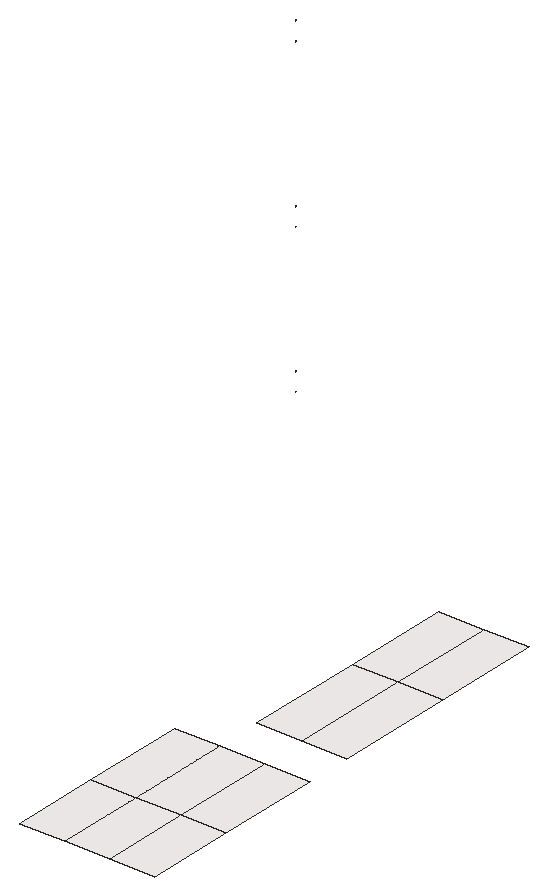
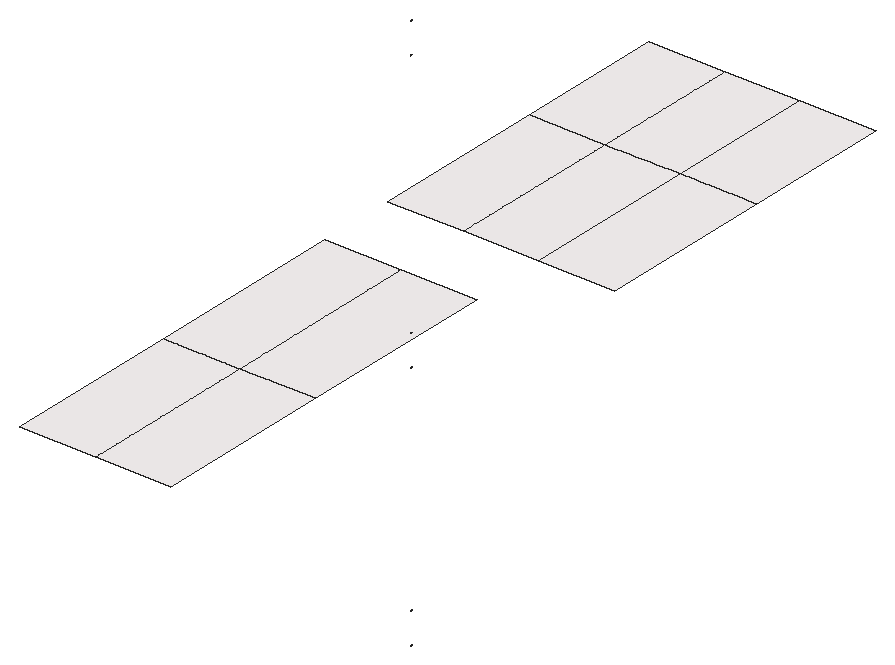
# SketchUp Ruby script. Lengths in inches.
U = 1.inch
M = Sketchup.active_model
def pt(a) = Geom::Point3d.new(a.map { |v| v * U })
def face(e, loops, mat)
  f = e.add_face(loops[0].map { |a| pt(a) })
  loops[1..].each { |l| e.add_face(l.map { |a| pt(a) }).erase! }
  f.material = f.back_material = mat if mat
  f
end
# faces: each face lists its corners as indices into pts; further lists are holes
def faces(e, pts, list, mat = nil) = list.each { |f| face(e, (f[0].is_a?(Array) ? f : [f]).map { |l| l.map { |i| pts[i] } }, mat) }
# xy, xz, yz: faces in a plane at the given z, y or x. An outline is a flat list of corners, or four numbers for a rectangle; further outlines are holes
def ring(l) = l.size == 4 ? [[l[0], l[1]], [l[2], l[1]], [l[2], l[3]], [l[0], l[3]]] : l.each_slice(2).to_a
def flat(e, list, mat, &to3) = list.each { |f| face(e, (f[0].is_a?(Array) ? f : [f]).map { |l| ring(l).map { |u, v| to3.(u, v) } }, mat) }
def xy(e, z, list, mat = nil) = flat(e, list, mat) { |x, y| [x, y, z] }
def xz(e, y, list, mat = nil) = flat(e, list, mat) { |x, z| [x, y, z] }
def yz(e, x, list, mat = nil) = flat(e, list, mat) { |y, z| [x, y, z] }
def lines(e, pts, list) = list.each { |a, b| e.add_line(pt(pts[a]), pt(pts[b])) }
# prism: a flat outline (further loops are holes) pulled along v
def prism(e, loops, v, mat = nil)
  f = face(e, loops, mat); d = Geom::Vector3d.new(v.map { |x| x * U })
  f.pushpull(f.normal.samedirection?(d) ? d.length : -d.length)
end
def box(e, o, s, mat = nil) = prism(e, [[o, [o[0] + s[0], o[1], o[2]], [o[0] + s[0], o[1] + s[1], o[2]], [o[0], o[1] + s[1], o[2]]]], [0, 0, s[2]], mat)
def at(x, y, z, deg = 0) = Geom::Transformation.translation(pt([x, y, z])) * Geom::Transformation.rotation(ORIGIN, Z_AXIS, deg.degrees)
def axes(o, x, y, z) = Geom::Transformation.new([*x, 0, *y, 0, *z, 0, *pt(o).to_a, 1])
def part(name) = M.definitions.add(name)
# library, detail: a bought-in or finely detailed component or shape, given as its bounding box
def library(name, o, s) = part(name).tap { |d| box(d.entities, o, s) }
def detail(e, o, s) = box(e.add_group.entities, o, s)
def put(e, d, t, mat = nil) = e.add_instance(d, t).tap { |i| i.material = mat if mat }
def group(e, t, mat = nil) = e.add_group.tap { |g| g.transformation = t; g.material = mat if mat }.entities
root = M.entities
M.materials.add("Material \#1").color = [140, 140, 140]
M.materials.add("[0010_Snow]").color = [255, 250, 250]
c1 = part("3DGeom~8_Defintion")
xz(c1.entities,-471.94,[[458.125,-17.29,459.53,-16.11,457.73,-17.15],[458.125,-17.29,458.54,-17.29,459.53,-16.11],[458.54,-17.29,458.93,-17.15,459.53,-16.11],[457.73,-17.15,459.53,-16.11,457.42,-16.88],[458.93,-17.15,459.25,-16.88,459.53,-16.11],
  [457.42,-16.88,459.53,-16.11,457.21,-16.52],[459.25,-16.88,459.46,-16.52,459.53,-16.11],[457.21,-16.52,459.53,-16.11,457.14,-16.11],[457.14,-16.11,459.53,-16.11,457.21,-15.7],[459.53,-16.11,457.42,-15.34,457.21,-15.7],
  [459.53,-16.11,457.73,-15.07,457.42,-15.34],[459.53,-16.11,458.125,-14.93,457.73,-15.07],[459.53,-16.11,458.54,-14.93,458.125,-14.93],[459.53,-16.11,458.93,-15.07,458.54,-14.93],[459.53,-16.11,459.25,-15.34,458.93,-15.07],
  [459.53,-16.11,459.46,-15.7,459.25,-15.34]],"Material \#1")
xz(c1.entities,-416.39,[[458.125,-17.29,457.73,-17.15,459.53,-16.11],[458.125,-17.29,459.53,-16.11,458.54,-17.29],[458.54,-17.29,459.53,-16.11,458.93,-17.15],[457.73,-17.15,457.42,-16.88,459.53,-16.11],[458.93,-17.15,459.53,-16.11,459.25,-16.88],
  [457.42,-16.88,457.21,-16.52,459.53,-16.11],[459.25,-16.88,459.53,-16.11,459.46,-16.52],[457.21,-16.52,457.14,-16.11,459.53,-16.11],[457.14,-16.11,457.21,-15.7,459.53,-16.11],[459.53,-16.11,457.21,-15.7,457.42,-15.34],
  [459.53,-16.11,457.42,-15.34,457.73,-15.07],[459.53,-16.11,457.73,-15.07,458.125,-14.93],[459.53,-16.11,458.125,-14.93,458.54,-14.93],[459.53,-16.11,458.54,-14.93,458.93,-15.07],[459.53,-16.11,458.93,-15.07,459.25,-15.34],
  [459.53,-16.11,459.25,-15.34,459.46,-15.7]],"Material \#1")
xz(c1.entities,-27.5,[[458.125,-17.29,459.53,-16.11,457.73,-17.15],[458.125,-17.29,458.54,-17.29,459.53,-16.11],[458.54,-17.29,458.93,-17.15,459.53,-16.11],[457.73,-17.15,459.53,-16.11,457.42,-16.88],[458.93,-17.15,459.25,-16.88,459.53,-16.11],
  [457.42,-16.88,459.53,-16.11,457.21,-16.52],[459.25,-16.88,459.46,-16.52,459.53,-16.11],[457.21,-16.52,459.53,-16.11,457.14,-16.11],[457.14,-16.11,459.53,-16.11,457.21,-15.7],[459.53,-16.11,457.42,-15.34,457.21,-15.7],
  [459.53,-16.11,457.73,-15.07,457.42,-15.34],[459.53,-16.11,458.125,-14.93,457.73,-15.07],[459.53,-16.11,458.54,-14.93,458.125,-14.93],[459.53,-16.11,458.93,-15.07,458.54,-14.93],[459.53,-16.11,459.25,-15.34,458.93,-15.07],
  [459.53,-16.11,459.46,-15.7,459.25,-15.34]],"Material \#1")
xz(c1.entities,28.06,[[458.125,-17.29,457.73,-17.15,459.53,-16.11],[458.125,-17.29,459.53,-16.11,458.54,-17.29],[458.54,-17.29,459.53,-16.11,458.93,-17.15],[457.73,-17.15,457.42,-16.88,459.53,-16.11],[458.93,-17.15,459.53,-16.11,459.25,-16.88],
  [457.42,-16.88,457.21,-16.52,459.53,-16.11],[459.25,-16.88,459.53,-16.11,459.46,-16.52],[457.21,-16.52,457.14,-16.11,459.53,-16.11],[457.14,-16.11,457.21,-15.7,459.53,-16.11],[459.53,-16.11,457.21,-15.7,457.42,-15.34],
  [459.53,-16.11,457.42,-15.34,457.73,-15.07],[459.53,-16.11,457.73,-15.07,458.125,-14.93],[459.53,-16.11,458.125,-14.93,458.54,-14.93],[459.53,-16.11,458.54,-14.93,458.93,-15.07],[459.53,-16.11,458.93,-15.07,459.25,-15.34],
  [459.53,-16.11,459.25,-15.34,459.46,-15.7]],"Material \#1")
xz(c1.entities,472.5,[[458.125,-17.29,459.53,-16.11,457.73,-17.15],[458.125,-17.29,458.54,-17.29,459.53,-16.11],[458.54,-17.29,458.93,-17.15,459.53,-16.11],[457.73,-17.15,459.53,-16.11,457.42,-16.88],[458.93,-17.15,459.25,-16.88,459.53,-16.11],
  [457.42,-16.88,459.53,-16.11,457.21,-16.52],[459.25,-16.88,459.46,-16.52,459.53,-16.11],[457.21,-16.52,459.53,-16.11,457.14,-16.11],[457.14,-16.11,459.53,-16.11,457.21,-15.7],[459.53,-16.11,457.42,-15.34,457.21,-15.7],
  [459.53,-16.11,457.73,-15.07,457.42,-15.34],[459.53,-16.11,458.125,-14.93,457.73,-15.07],[459.53,-16.11,458.54,-14.93,458.125,-14.93],[459.53,-16.11,458.93,-15.07,458.54,-14.93],[459.53,-16.11,459.25,-15.34,458.93,-15.07],
  [459.53,-16.11,459.46,-15.7,459.25,-15.34]],"Material \#1")
xz(c1.entities,528.06,[[458.125,-17.29,457.73,-17.15,459.53,-16.11],[458.125,-17.29,459.53,-16.11,458.54,-17.29],[458.54,-17.29,459.53,-16.11,458.93,-17.15],[457.73,-17.15,457.42,-16.88,459.53,-16.11],[458.93,-17.15,459.53,-16.11,459.25,-16.88],
  [457.42,-16.88,457.21,-16.52,459.53,-16.11],[459.25,-16.88,459.53,-16.11,459.46,-16.52],[457.21,-16.52,457.14,-16.11,459.53,-16.11],[457.14,-16.11,457.21,-15.7,459.53,-16.11],[459.53,-16.11,457.21,-15.7,457.42,-15.34],
  [459.53,-16.11,457.42,-15.34,457.73,-15.07],[459.53,-16.11,457.73,-15.07,458.125,-14.93],[459.53,-16.11,458.125,-14.93,458.54,-14.93],[459.53,-16.11,458.54,-14.93,458.93,-15.07],[459.53,-16.11,458.93,-15.07,459.25,-15.34],
  [459.53,-16.11,459.25,-15.34,459.46,-15.7]],"Material \#1")
xy(root,-7.5625,[[415.5625,6.25,427.5625,29.875],[427.5625,6.25,439.5625,29.875],[439.5625,6.25,451.5625,29.875],[415.5625,29.875,427.5625,57.9375],[427.5625,29.875,439.5625,57.9375],
  [439.5625,29.875,451.5625,57.9375],[427.5625,70.375,439.5625,102.3125],[439.5625,70.375,451.5625,102.3125],[427.5625,102.3125,439.5625,130.875],[439.5625,102.3125,451.5625,130.875]],"[0010_Snow]")
put(root,c1,axes([362.67,201.8,49.3125],[0,-0.08145,0],[0,0,0.08876],[0.0037,0,0]),"Material \#1")
